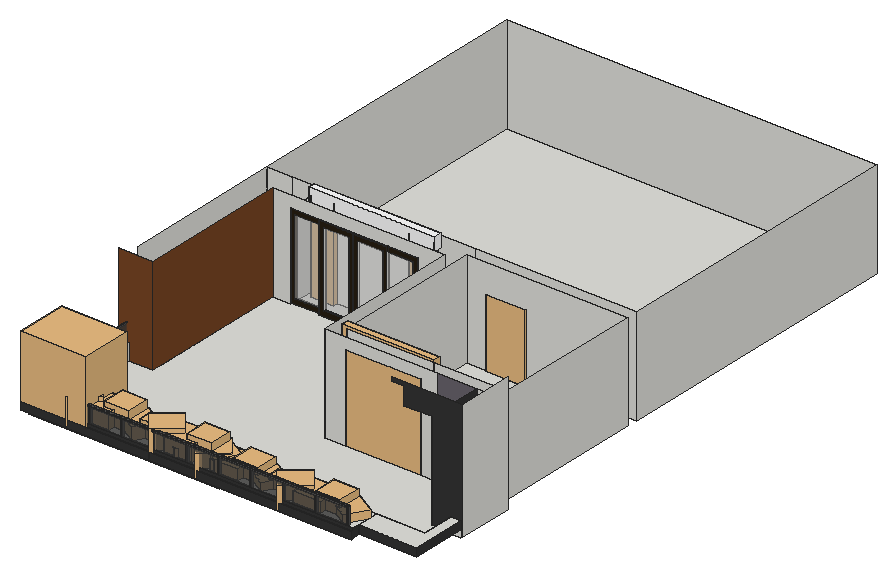
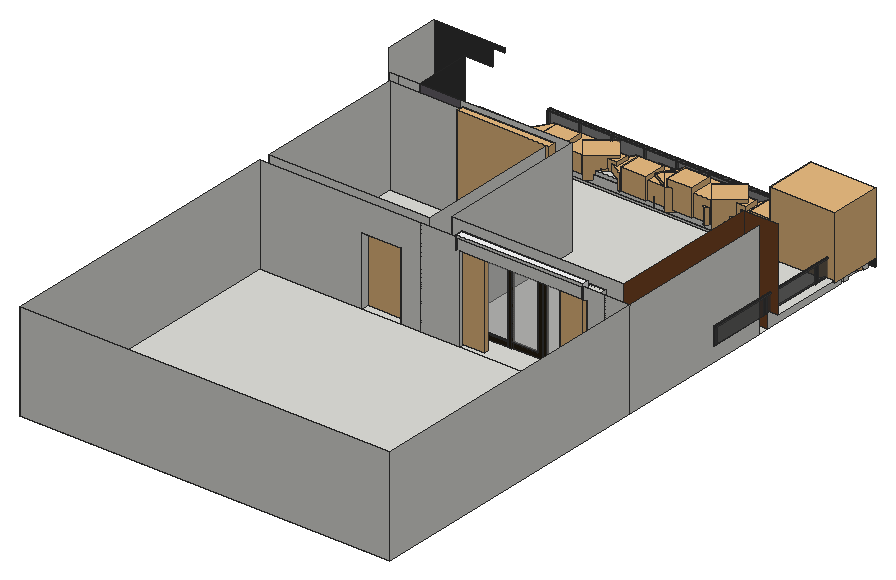
# SketchUp Ruby script. Lengths in inches.
U = 1.inch
M = Sketchup.active_model
def pt(a) = Geom::Point3d.new(a.map { |v| v * U })
def face(e, loops, mat)
  f = e.add_face(loops[0].map { |a| pt(a) })
  loops[1..].each { |l| e.add_face(l.map { |a| pt(a) }).erase! }
  f.material = f.back_material = mat if mat
  f
end
# faces: each face lists its corners as indices into pts; further lists are holes
def faces(e, pts, list, mat = nil) = list.each { |f| face(e, (f[0].is_a?(Array) ? f : [f]).map { |l| l.map { |i| pts[i] } }, mat) }
# xy, xz, yz: faces in a plane at the given z, y or x. An outline is a flat list of corners, or four numbers for a rectangle; further outlines are holes
def ring(l) = l.size == 4 ? [[l[0], l[1]], [l[2], l[1]], [l[2], l[3]], [l[0], l[3]]] : l.each_slice(2).to_a
def flat(e, list, mat, &to3) = list.each { |f| face(e, (f[0].is_a?(Array) ? f : [f]).map { |l| ring(l).map { |u, v| to3.(u, v) } }, mat) }
def xy(e, z, list, mat = nil) = flat(e, list, mat) { |x, y| [x, y, z] }
def xz(e, y, list, mat = nil) = flat(e, list, mat) { |x, z| [x, y, z] }
def yz(e, x, list, mat = nil) = flat(e, list, mat) { |y, z| [x, y, z] }
def lines(e, pts, list) = list.each { |a, b| e.add_line(pt(pts[a]), pt(pts[b])) }
# prism: a flat outline (further loops are holes) pulled along v
def prism(e, loops, v, mat = nil)
  f = face(e, loops, mat); d = Geom::Vector3d.new(v.map { |x| x * U })
  f.pushpull(f.normal.samedirection?(d) ? d.length : -d.length)
end
def box(e, o, s, mat = nil) = prism(e, [[o, [o[0] + s[0], o[1], o[2]], [o[0] + s[0], o[1] + s[1], o[2]], [o[0], o[1] + s[1], o[2]]]], [0, 0, s[2]], mat)
def at(x, y, z, deg = 0) = Geom::Transformation.translation(pt([x, y, z])) * Geom::Transformation.rotation(ORIGIN, Z_AXIS, deg.degrees)
def axes(o, x, y, z) = Geom::Transformation.new([*x, 0, *y, 0, *z, 0, *pt(o).to_a, 1])
def part(name) = M.definitions.add(name)
# library, detail: a bought-in or finely detailed component or shape, given as its bounding box
def library(name, o, s) = part(name).tap { |d| box(d.entities, o, s) }
def detail(e, o, s) = box(e.add_group.entities, o, s)
def put(e, d, t, mat = nil) = e.add_instance(d, t).tap { |i| i.material = mat if mat }
def group(e, t, mat = nil) = e.add_group.tap { |g| g.transformation = t; g.material = mat if mat }.entities
root = M.entities
M.materials.add("DefaultMaterial4").color = [255, 255, 255]
M.materials.add("Material__1").color = [95, 70, 46]
M.materials.add("[0135_DarkGray]").color = [81, 81, 81]
M.materials.add("[Color M07]").color = [53, 53, 53]
M.materials.add("[Slate Light Tile]").color = [105, 101, 109]
M.materials.add("[Translucent Glass Gray]2").color = [201, 201, 201]
M.materials["[Translucent Glass Gray]2"].alpha = 0.5
M.materials.add("[Translucent Glass Safety]").color = [204, 235, 244]
M.materials["[Translucent Glass Safety]"].alpha = 0.5
M.materials.add("[Translucent_Glass_Gray]1").color = [63, 63, 63]
M.materials["[Translucent_Glass_Gray]1"].alpha = 0.54
M.materials.add("[Wood Veneer 01]").color = [120, 70, 37]
M.materials.add("curtain").color = [207, 207, 207]
M.materials["curtain"].alpha = 0.74
M.materials.add("oak swatch").color = [40, 31, 19]
c1 = library("Group\#21",[-0.5,-0.5,0],[11,185.21,2.6875])
c2 = library("Mesh Light\#2",[-0.5,-0.5,-0.1],[1,1,0.2])
c3 = library("Group\#22",[-0.5,-0.5,-0.1],[11,185.21,0.2])
c4 = library("Group\#20",[-0.5,-0.5,-0.1],[11,185.21,0.2])
c5 = library("元件\#5",[-4.39,0,0],[5.37,35.83,90.55])
c6 = library("Sliding Door",[0,0,0],[94.49,5.83,91.73])
c7 = part("Group\#1")
box(c7.entities,[0,0,0],[1.77,4.72,80.31],"oak swatch")
c8 = part("Exterior Sliding Doors")
xy(c8.entities,0,[[1.77,33.07,3.54,70.87],[1.77,70.87,3.54,108.66]])
xy(c8.entities,0,[[0,0,1.77,33.07],[0,108.66,1.77,141.73]],"oak swatch")
xy(c8.entities,4.72,[[0,4.72,1.77,33.07],[1.77,37.8,3.54,66.14],[1.77,75.88,3.54,103.9375],[0,108.66,1.77,137.01]],"oak swatch")
xy(c8.entities,75.59,[[1.77,37.8,3.54,66.14],[1.77,75.88,3.54,103.9375]])
xy(c8.entities,75.59,[[0,4.72,1.77,33.07],[0,108.66,1.77,137.01]],"oak swatch")
xy(c8.entities,80.31,[[0,0,1.77,33.07],[1.77,33.07,3.54,70.87],[1.77,70.87,3.54,108.66],[0,108.66,1.77,141.73]],"oak swatch")
xz(c8.entities,0,[[0,0,1.77,80.31]],"oak swatch")
xz(c8.entities,4.72,[[0,4.72,1.77,75.59]],"oak swatch")
xz(c8.entities,33.07,[[0,0,1.77,4.72],[1.77,0,3.54,80.31],[0,75.59,1.77,80.31]],"oak swatch")
xz(c8.entities,37.8,[[1.77,4.72,3.54,75.59]])
xz(c8.entities,66.14,[[1.77,4.72,3.54,75.59]],"oak swatch")
xz(c8.entities,70.87,[[1.77,0,3.54,80.31]])
xz(c8.entities,75.88,[[1.77,4.72,3.54,75.59]])
xz(c8.entities,103.9375,[[1.77,4.72,3.54,75.59]],"oak swatch")
xz(c8.entities,108.66,[[1.77,4.72,3.54,75.59]])
xz(c8.entities,108.66,[[0,0,3.54,4.72],[0,75.59,3.54,80.31]],"oak swatch")
xz(c8.entities,137.01,[[0,4.72,1.77,75.59]],"oak swatch")
xz(c8.entities,141.73,[[0,0,1.77,80.31]],"oak swatch")
yz(c8.entities,0,[[0,0,33.07,0,33.07,4.72,4.72,4.72,4.72,75.59,33.07,75.59,33.07,80.31,0,80.31],[108.66,0,141.73,0,141.73,80.31,108.66,80.31,108.66,75.59,137.01,75.59,137.01,4.72,108.66,4.72]],"oak swatch")
yz(c8.entities,1.77,[[4.72,4.72,33.07,75.59],[37.8,4.72,66.14,75.59],[75.88,4.72,103.9375,75.59],[108.66,4.72,137.01,75.59]],"[Translucent Glass Gray]2")
yz(c8.entities,1.77,[[0,0,33.07,0,33.07,4.72,4.72,4.72,4.72,75.59,33.07,75.59,33.07,80.31,0,80.31],[[33.07,0,70.87,80.31],[37.8,4.72,66.14,75.59]],[[70.87,0,141.73,80.31],[108.66,4.72,137.01,75.59],[75.88,4.72,103.9375,75.59]]],"oak swatch")
yz(c8.entities,3.54,[[[33.07,0,70.87,80.31],[37.8,4.72,66.14,75.59]],[[70.87,0,108.66,80.31],[75.88,4.72,103.9375,75.59]]],"oak swatch")
put(c8.entities,c7,at(0,33.07,0))
put(c8.entities,c7,at(0,103.9375,0))
c9 = library("Plane02",[0.84,-3.92,-95.52],[32.2,7.84,95.63])
c10 = library("Window curtains",[0,0,0],[5.91,79.92,51.3])
c11 = library("Areca palm plant",[0,0,0],[49.1,36.6,54.46])
c12 = library("Group38\#2",[14.01,28.44,-23.43],[18.58,18.32,38.89])
c13 = library("Group\#32",[-84.69,-90.07,-0.36],[176.51,175.13,171.4])
c14 = library("Group20\#1",[-20.81,-17.08,3.79],[39.86,39.43,37.51])
c15 = library("Group\#130",[-7.34,-1.2,0],[38.67,35.81,49.04])
c16 = part("Group\#35")
put(c16.entities,c11,axes([-6.2,158.41,6.08],[0.45017,-0.56191,0],[0.66137,0.52986,0],[0,0,0.72]))
put(c16.entities,c11,axes([-6.2,56.6,6.08],[0.45017,-0.56191,0],[0.66137,0.52986,0],[0,0,0.72]))
put(c16.entities,c12,axes([-4.1,-1.15,28.17],[0.8848,0,0],[0,0.94674,0],[0,0,0.85826]))
put(c16.entities,c12,axes([-4.1,100.66,28.17],[0.8848,0,0],[0,0.94674,0],[0,0,0.85826]))
g1 = group(c16.entities,at(0,0,0))
xy(g1,0,[[0,0,6,234.8],[30,0,36,234.8]])
xy(g1,3,[[6,0,30,234.8]])
xy(g1,7,[[6,5,30,229.8]],"Material__1")
xy(g1,15,[[[0,0,36,234.8],[6,5,30,229.8]]])
xz(g1,0,[[0,0,6,0,6,3,30,3,30,0,36,0,36,15,0,15]])
xz(g1,5,[[6,7,30,15]])
xz(g1,229.8,[[6,7,30,15]])
xz(g1,234.8,[[0,0,0,15,36,15,36,0,30,0,30,3,6,3,6,0]])
yz(g1,0,[[0,0,234.8,15]])
yz(g1,6,[[0,0,234.8,3],[5,7,229.8,15]])
yz(g1,30,[[0,0,234.8,3],[5,7,229.8,15]])
yz(g1,36,[[0,0,234.8,15]])
put(c16.entities,c13,axes([17.19,121.23,6.07],[-0.08133,-0.14087,0],[0.14087,-0.08133,0],[0,0,0.1725]))
put(c16.entities,c13,axes([14.93,173.12,6.05],[-0.04961,-0.08593,0],[0.08593,-0.04961,0],[0,0,0.10522]))
put(c16.entities,c14,axes([18.97,79.98,4.77],[0,0.85,0],[-0.85,0,0],[0,0,0.85]))
put(c16.entities,c13,axes([17.19,223.04,6.07],[-0.08133,-0.14087,0],[0.14087,-0.08133,0],[0,0,0.1725]))
put(c16.entities,c13,axes([14.93,71.3,6.05],[-0.04961,-0.08593,0],[0.08593,-0.04961,0],[0,0,0.10522]))
put(c16.entities,c15,axes([24.9375,191.72,8],[0,0.79,0],[-0.79,0,0],[0,0,0.79]))
put(c16.entities,c14,axes([18.97,181.79,4.77],[0,0.85,0],[-0.85,0,0],[0,0,0.85]))
put(c16.entities,c15,axes([24.9375,89.91,8],[0,0.79,0],[-0.79,0,0],[0,0,0.79]))
put(c16.entities,c13,axes([14.93,91.37,6.05],[-0.04961,-0.08593,0],[0.08593,-0.04961,0],[0,0,0.10522]))
put(c16.entities,c13,axes([14.93,145.87,6.05],[-0.04961,-0.08593,0],[0.08593,-0.04961,0],[0,0,0.10522]))
put(c16.entities,c13,axes([17.19,15.79,6.07],[-0.08133,-0.14087,0],[0.14087,-0.08133,0],[0,0,0.1725]))
put(c16.entities,c13,axes([14.93,193.18,6.05],[-0.04961,-0.08593,0],[0.08593,-0.04961,0],[0,0,0.10522]))
put(c16.entities,c13,axes([14.93,44.05,6.05],[-0.04961,-0.08593,0],[0.08593,-0.04961,0],[0,0,0.10522]))
c17 = library("Round Planter with Plant",[-35.48,-39.77,0],[80.62,63.55,77.875])
c18 = part("Group\#81")
box(c18.entities,[0,0,0],[0.79,39.37,35.43],"[Translucent_Glass_Gray]1")
c19 = part("Group\#82")
box(c19.entities,[0,0,0],[0.59,1.57,34.25])
c20 = part("Group\#85")
g2 = group(c20.entities,at(0.55,0.5,0))
put(g2,c18,axes([293.06,0,0],[0,0.84,0],[-0.92977,0,0],[0,0,1]),"[Translucent Glass Safety]")
g3 = group(g2,at(0,33.57,0),"[Translucent Glass Safety]")
box(g3,[0,0,0],[0.73,33.07,35.43],"[Translucent_Glass_Gray]1")
put(g2,c18,axes([218.38,0,0],[0,0.84,0],[-0.92977,0,0],[0,0,1]),"[Translucent Glass Safety]")
put(g2,c18,axes([367.73,0,0],[0,0.84,0],[-0.92977,0,0],[0,0,1]),"[Translucent Glass Safety]")
g4 = group(g2,at(31.69,0,0),"[Translucent Glass Safety]")
box(g4,[-30.96,0,0],[30.96,0.66,35.43],"[Translucent_Glass_Gray]1")
put(g2,c18,axes([255.72,0,0],[0,0.84,0],[-0.92977,0,0],[0,0,1]),"[Translucent Glass Safety]")
g5 = group(g2,at(181.04,0,0),"[Translucent Glass Safety]")
box(g5,[-36.61,0,0],[36.61,0.66,35.43],"[Translucent_Glass_Gray]1")
g6 = group(g2,at(0,0.66,0),"[Translucent Glass Safety]")
box(g6,[0,0,0],[0.73,32.24,35.43],"[Translucent_Glass_Gray]1")
g7 = group(g2,at(143.71,0,0),"[Translucent Glass Safety]")
box(g7,[-36.61,0,0],[36.61,0.66,35.43],"[Translucent_Glass_Gray]1")
g8 = group(g2,at(69.03,0,0),"[Translucent Glass Safety]")
box(g8,[-36.61,0,0],[36.61,0.66,35.43],"[Translucent_Glass_Gray]1")
g9 = group(g2,at(0,67.3,0),"[Translucent Glass Safety]")
box(g9,[0,0,0],[0.73,33.07,35.43],"[Translucent_Glass_Gray]1")
put(g2,c19,axes([107.44,0.66,0],[0,1,0],[-0.92977,0,0],[0,0,1]),"[0135_DarkGray]")
put(g2,c19,axes([144.78,0.66,0],[0,1,0],[-0.92977,0,0],[0,0,1]),"[0135_DarkGray]")
put(g2,c19,axes([182.11,0.66,0],[0,1,0],[-0.92977,0,0],[0,0,1]),"[0135_DarkGray]")
put(g2,c19,axes([256.79,0.66,0],[0,1,0],[-0.92977,0,0],[0,0,1]),"[0135_DarkGray]")
put(g2,c19,axes([368.14,0.66,0],[0,1,0],[-0.92977,0,0],[0,0,1]),"[0135_DarkGray]")
put(g2,c19,axes([0.73,98.83,0],[0.92977,0,0],[0,1,0],[0,0,1]),"[0135_DarkGray]")
put(g2,c19,axes([331.46,0.66,0],[0,1,0],[-0.92977,0,0],[0,0,1]),"[0135_DarkGray]")
g10 = group(g2,at(106.37,0,0),"[Translucent Glass Safety]")
box(g10,[-36.61,0,0],[36.61,0.66,35.43],"[Translucent_Glass_Gray]1")
put(g2,c18,axes([330.39,0,0],[0,0.84,0],[-0.92977,0,0],[0,0,1]),"[Translucent Glass Safety]")
put(g2,c19,axes([294.125,0.66,0],[0,1,0],[-0.92977,0,0],[0,0,1]),"[0135_DarkGray]")
put(g2,c19,axes([0.73,66.04,0],[0.92977,0,0],[0,1,0],[0,0,1]),"[0135_DarkGray]")
put(g2,c19,axes([0.73,32.31,0],[0.92977,0,0],[0,1,0],[0,0,1]),"[0135_DarkGray]")
put(g2,c19,axes([32.76,0.66,0],[0,1,0],[-0.92977,0,0],[0,0,1]),"[0135_DarkGray]")
put(g2,c19,axes([70.1,0.66,0],[0,1,0],[-0.92977,0,0],[0,0,1]),"[0135_DarkGray]")
put(g2,c19,axes([219.45,0.66,0],[0,1,0],[-0.92977,0,0],[0,0,1]),"[0135_DarkGray]")
g11 = group(c20.entities,at(0,0,34.25))
xy(g11,0,[[0,0,0,100.87,0.55,100.87,0.55,0.5,362.73,0.5,362.73,0],[362.73,0,369.35,0.5],[368.19,0.5,368.6875,1.16],[1.28,1.16,1.28,100.87,1.83,100.87,1.83,1.65,362.73,1.65,362.73,1.16],[362.73,1.16,368.19,1.65]],"[0135_DarkGray]")
xy(g11,1.18,[[368.19,0,368.6875,0.5],[368.6875,0,369.35,0.5],[0.55,0.5,0.55,100.87,1.28,100.87,1.28,1.16,362.73,1.16,362.73,0.5],[368.6875,0.5,369.35,1.16]],"[0135_DarkGray]")
xy(g11,1.97,[[0,0,362.73,0,362.73,1.65,1.83,1.65,1.83,100.87,0,100.87],[362.73,0,368.19,1.65]],"[0135_DarkGray]")
xz(g11,0,[[0,0,362.73,1.97],[362.73,0,369.35,0,369.35,1.18,368.19,1.18,368.19,1.97,362.73,1.97]],"[0135_DarkGray]")
xz(g11,0.5,[[0.55,0,1.28,1.18],[1.28,0,362.73,1.18],[362.73,0,368.19,1.18],[368.19,0,368.6875,1.18],[368.6875,0,369.35,1.18]],"[0135_DarkGray]")
xz(g11,1.16,[[1.28,0,362.73,1.18],[362.73,0,368.19,1.18]],"[0135_DarkGray]")
xz(g11,1.65,[[1.83,0,362.73,1.97],[362.73,0,368.19,1.97]],"[0135_DarkGray]")
xz(g11,100.87,[[0,0,0,1.97,1.83,1.97,1.83,0,1.28,0,1.28,1.18,0.55,1.18,0.55,0]],"[0135_DarkGray]")
yz(g11,0,[[0,0,100.87,1.97]],"[0135_DarkGray]")
yz(g11,0.55,[[0.5,0,100.87,1.18]],"[0135_DarkGray]")
yz(g11,1.28,[[1.16,0,100.87,1.18]],"[0135_DarkGray]")
yz(g11,1.83,[[1.65,0,100.87,1.97]],"[0135_DarkGray]")
yz(g11,362.73,[[0,0,0,1.97,1.65,1.97,1.65,0,1.16,0,1.16,1.18,0.5,1.18,0.5,0]],"[0135_DarkGray]")
yz(g11,368.19,[[1.16,0,1.65,0,1.65,1.97,0,1.97,0,1.18,1.16,1.18],[0.5,0,1.16,1.18]],"[0135_DarkGray]")
yz(g11,368.6875,[[0.5,0,1.16,1.18]],"[0135_DarkGray]")
yz(g11,369.35,[[0,0,0.5,1.18]],"[0135_DarkGray]")
c21 = library("Spot Light",[-5.1,-5.1,-11.05],[10.2,10.2,11.05])
c22 = part("Group\#68")
xy(c22.entities,48.43,[[59.06,0,59.06,5.91,59.65,5.91,59.65,0.59,138.39,0.59,138.39,5.91,138.98,5.91,138.98,0]],"DefaultMaterial4")
xy(c22.entities,53.9375,[[59.65,0.59,138.39,5.91]],"DefaultMaterial4")
xy(c22.entities,55.51,[[59.06,0,138.98,5.91]],"DefaultMaterial4")
xz(c22.entities,0,[[59.06,48.43,138.98,55.51]],"DefaultMaterial4")
xz(c22.entities,0.59,[[59.65,48.43,138.39,53.9375]],"DefaultMaterial4")
xz(c22.entities,5.91,[[59.06,48.43,59.06,55.51,138.98,55.51,138.98,48.43,138.39,48.43,138.39,53.9375,59.65,53.9375,59.65,48.43]])
yz(c22.entities,59.06,[[0,48.43,5.91,55.51]],"DefaultMaterial4")
yz(c22.entities,138.39,[[0.59,48.43,5.91,53.9375]],"DefaultMaterial4")
yz(c22.entities,138.98,[[0,48.43,5.91,55.51]],"DefaultMaterial4")
xy(root,132,[[190.19,395.75,645.31,395.75,645.31,438.56,619.25,438.56,619.25,508.37,550.28,508.37,550.28,522.1,457.97,522.1,457.97,508.37,431.89,508.37,431.89,692.93,399.32,692.93,399.32,721.37,242.57,721.37,242.57,692.93,220.4375,692.93,220.4375,508.37,190.19,508.37],[645.31,436.28,657.75,438.56],[619.25,438.56,657.75,508.37],[190.19,508.37,220.4375,522.1],[190.19,522.1,220.4375,522.1,220.4375,692.93,220.5,692.93,220.5,721.37,190.19,721.37],
  [447.875,522.1,645.31,522.1,645.31,707.71,519.83,707.71,519.83,721.37,471.83,721.37,471.83,707.71,447.875,707.71],[190.19,721.37,645.31,1090.87]])
xy(root,139.1,[[177.75,357.25,585.62,359.375]])
xy(root,141.4375,[[585.62,368.125,585.62,395.75,645.31,395.75,645.31,436.28,657.75,436.28,657.75,368.125]])
xy(root,148.36,[[177.75,357.25,585.62,359.375]])
xy(root,151.5,[[177.75,359.375,585.62,359.375,585.62,395.75,190.19,395.75,190.19,508.37,177.75,508.37],[585.62,368.125,657.75,368.125,657.75,436.28,645.31,436.28,645.31,395.75,585.62,395.75]])
xy(root,195.89,[[590.91,497.87,596.29,508.37]])
xy(root,212.71,[[590.91,497.87,596.29,508.37]])
xy(root,216,[[471.83,707.71,519.83,721.37]])
xy(root,237.9375,[[242.57,692.93,399.32,721.37]])
xy(root,238.0625,[[457.97,508.37,550.28,522.1]])
xz(root,357.25,[[177.75,139.1,585.62,148.36]],"[Color M07]")
xz(root,359.375,[[177.75,148.36,585.62,151.5]],"[Color M07]")
xz(root,368.125,[[585.62,141.4375,657.75,151.5]],"[Color M07]")
xz(root,395.75,[[190.19,132,585.62,151.5],[585.62,132,645.31,141.4375],[585.62,141.4375,645.31,151.5]])
xz(root,436.28,[[645.31,132,657.75,141.4375],[645.31,141.4375,657.75,151.5]])
xz(root,438.56,[[619.25,132,657.75,132,657.75,278.125,569.82,278.125,569.82,273.1875,585.62,273.1875,585.62,252,619.25,252]],"[Color M07]")
xz(root,497.87,[[590.91,195.89,596.29,212.71]])
xz(root,508.37,[[431.89,132,457.97,132,457.97,238.0625,550.28,238.0625,550.28,132,569.82,132,569.82,252,431.89,252],[619.25,132,645.31,252],[645.31,132,657.75,252]])
xz(root,508.37,[[[569.82,132,619.25,252],[590.91,195.89,596.29,212.71]]],"[Slate Light Tile]")
xz(root,508.37,[[190.19,132,220.4375,132,220.4375,252,177.75,252,177.75,151.5,190.19,151.5]],"[Wood Veneer 01]")
xz(root,522.1,[[447.875,132,447.875,252,645.31,252,645.31,132,550.28,132,550.28,238.0625,457.97,238.0625,457.97,132]])
xz(root,692.93,[[220.4375,132,242.57,132,242.57,237.9375,399.32,237.9375,399.32,132,431.89,132,431.89,252,220.4375,252]])
xz(root,707.71,[[447.875,132,471.83,132,471.83,216,519.83,216,519.83,132,645.31,132,645.31,252,447.875,252]])
xz(root,721.37,[[190.19,132,220.5,252],[220.5,132,220.5,252,447.875,252,447.875,132,399.32,132,399.32,237.9375,242.57,237.9375,242.57,132],[447.875,132,447.875,252,645.31,252,645.31,132,519.83,132,519.83,216,471.83,216,471.83,132]])
xz(root,1090.87,[[190.19,132,645.31,252]])
yz(root,190.19,[[395.75,132,508.37,151.5],[522.1,132,721.37,252],[721.37,132,1090.87,252]])
yz(root,220.4375,[[508.37,132,692.93,252]],"[Wood Veneer 01]")
yz(root,242.57,[[692.93,132,721.37,237.9375]])
yz(root,399.32,[[692.93,132,721.37,237.9375]])
yz(root,431.89,[[508.37,132,692.93,252]])
yz(root,447.875,[[522.1,132,707.71,252]])
yz(root,457.97,[[508.37,132,522.1,238.0625]])
yz(root,471.83,[[707.71,132,721.37,216]])
yz(root,519.83,[[707.71,132,721.37,216]])
yz(root,550.28,[[508.37,132,522.1,238.0625]])
yz(root,585.62,[[368.125,141.4375,395.75,151.5]])
yz(root,585.62,[[357.25,139.1,359.375,139.1,368.125,141.4375,368.125,151.5,359.375,151.5,359.375,148.36,357.25,148.36]],"[Color M07]")
yz(root,590.91,[[497.87,195.89,508.37,212.71]])
yz(root,596.29,[[497.87,195.89,508.37,212.71]])
yz(root,619.25,[[438.56,132,508.37,252]],"[Color M07]")
yz(root,645.31,[[395.75,132,436.28,141.4375],[522.1,132,707.71,252],[721.37,132,1090.87,252],[395.75,141.4375,436.28,151.5]])
yz(root,657.75,[[438.56,132,508.37,278.125]])
yz(root,657.75,[[368.125,141.4375,436.28,151.5]],"[Color M07]")
p = [[496.4,385.12,126],[495.11,385.29,126],[495.11,385.29,128.6875],[496.4,385.12,128.6875],[497.69,385.29,126],[497.69,385.29,128.6875],
  [552.71,385.12,126],[551.42,385.29,126],[551.42,385.29,128.6875],[552.71,385.12,128.6875],[554.01,385.29,126],[554.01,385.29,128.6875],
  [493.9,385.79,126],[493.9,385.79,128.6875],[498.9,385.79,126],[498.9,385.79,128.6875],[550.21,385.79,126],[550.21,385.79,128.6875],
  [555.21,385.79,126],[555.21,385.79,128.6875],[492.86,386.58,126],[492.86,386.58,128.6875],[499.93,386.58,126],[499.93,386.58,128.6875],
  [549.18,386.58,126],[549.18,386.58,128.6875],[556.25,386.58,126],[556.25,386.58,128.6875],[492.07,387.62,126],[492.07,387.62,128.6875],
  [500.73,387.62,126],[500.73,387.62,128.6875],[548.38,387.62,126],[548.38,387.62,128.6875],[557.04,387.62,126],[557.04,387.62,128.6875],
  [491.57,388.83,126],[491.57,388.83,128.6875],[501.23,388.83,126],[501.23,388.83,128.6875],[547.88,388.83,126],[547.88,388.83,128.6875],
  [557.54,388.83,126],[557.54,388.83,128.6875],[491.4,390.12,126],[491.4,390.12,128.6875],[501.4,390.12,126],[501.4,390.12,128.6875],
  [547.71,390.12,126],[547.71,390.12,128.6875],[557.71,390.12,126],[557.71,390.12,128.6875],[491.57,391.41,126],[491.57,391.41,128.6875],
  [501.23,391.41,126],[501.23,391.41,128.6875],[547.88,391.41,126],[547.88,391.41,128.6875],[557.54,391.41,126],[557.54,391.41,128.6875],
  [492.07,392.62,126],[492.07,392.62,128.6875],[500.73,392.62,126],[500.73,392.62,128.6875],[548.38,392.62,126],[548.38,392.62,128.6875],
  [557.04,392.62,126],[557.04,392.62,128.6875],[492.86,393.66,126],[492.86,393.66,128.6875],[499.93,393.66,126],[499.93,393.66,128.6875],
  [549.18,393.66,126],[549.18,393.66,128.6875],[556.25,393.66,126],[556.25,393.66,128.6875],[493.9,394.45,126],[493.9,394.45,128.6875],
  [498.9,394.45,126],[498.9,394.45,128.6875],[550.21,394.45,126],[550.21,394.45,128.6875],[555.21,394.45,126],[555.21,394.45,128.6875],
  [495.11,394.95,126],[495.11,394.95,128.6875],[497.69,394.95,126],[497.69,394.95,128.6875],[551.42,394.95,126],[551.42,394.95,128.6875],
  [554.01,394.95,126],[554.01,394.95,128.6875],[496.4,395.12,126],[496.4,395.12,128.6875],[552.71,395.12,126],[552.71,395.12,128.6875],
  [552.71,439.5625,126],[551.42,439.73,126],[551.42,439.73,128.6875],[552.71,439.5625,128.6875],[554.01,439.73,126],[554.01,439.73,128.6875],
  [550.21,440.23,126],[550.21,440.23,128.6875],[555.21,440.23,126],[555.21,440.23,128.6875],[549.18,441.03,126],[549.18,441.03,128.6875],
  [556.25,441.03,126],[556.25,441.03,128.6875],[548.38,442.0625,126],[548.38,442.0625,128.6875],[557.04,442.0625,126],[557.04,442.0625,128.6875],
  [547.88,443.27,126],[547.88,443.27,128.6875],[557.54,443.27,126],[557.54,443.27,128.6875],[547.71,444.5625,126],[547.71,444.5625,128.6875],
  [557.71,444.5625,126],[557.71,444.5625,128.6875],[547.88,445.86,126],[547.88,445.86,128.6875],[557.54,445.86,126],[557.54,445.86,128.6875],
  [548.38,447.0625,126],[548.38,447.0625,128.6875],[557.04,447.0625,126],[557.04,447.0625,128.6875],[549.18,448.1,126],[549.18,448.1,128.6875],
  [556.25,448.1,126],[556.25,448.1,128.6875],[550.21,448.89,126],[550.21,448.89,128.6875],[555.21,448.89,126],[555.21,448.89,128.6875],
  [551.42,449.39,126],[551.42,449.39,128.6875],[554.01,449.39,126],[554.01,449.39,128.6875],[552.71,449.5625,126],[552.71,449.5625,128.6875],
  [552.71,500.05,126],[551.42,500.22,126],[551.42,500.22,128.6875],[552.71,500.05,128.6875],[554.01,500.22,126],[554.01,500.22,128.6875],
  [550.21,500.72,126],[550.21,500.72,128.6875],[555.21,500.72,126],[555.21,500.72,128.6875],[549.18,501.52,126],[549.18,501.52,128.6875],
  [556.25,501.52,126],[556.25,501.52,128.6875],[548.38,502.55,126],[548.38,502.55,128.6875],[557.04,502.55,126],[557.04,502.55,128.6875],
  [547.88,503.76,126],[547.88,503.76,128.6875],[557.54,503.76,126],[557.54,503.76,128.6875],[547.71,505.05,126],[547.71,505.05,128.6875],
  [557.71,505.05,126],[557.71,505.05,128.6875],[547.88,506.35,126],[547.88,506.35,128.6875],[557.54,506.35,126],[557.54,506.35,128.6875],
  [548.38,507.55,126],[548.38,507.55,128.6875],[557.04,507.55,126],[557.04,507.55,128.6875],[499.93,508.59,126],[500.73,507.55,126],
  [500.73,507.55,128.125],[499.93,508.59,128.125],[549.18,508.59,126],[549.18,508.59,128.6875],[556.25,508.59,126],[556.25,508.59,128.6875],
  [498.9,509.38,126],[498.9,509.38,128.125],[550.21,509.38,126],[550.21,509.38,128.6875],[555.21,509.38,126],[555.21,509.38,128.6875],
  [497.69,509.88,126],[497.69,509.88,128.125],[551.42,509.88,126],[551.42,509.88,128.6875],[554.01,509.88,126],[554.01,509.88,128.6875],
  [496.4,510.05,126],[496.4,510.05,128.125],[552.71,510.05,126],[552.71,510.05,128.6875],[552.71,559.33,126],[551.42,559.5,126],
  [551.42,559.5,128.6875],[552.71,559.33,128.6875],[554.01,559.5,126],[554.01,559.5,128.6875],[550.21,560,126],[550.21,560,128.6875],
  [555.21,560,126],[555.21,560,128.6875],[549.18,560.79,126],[549.18,560.79,128.6875],[556.25,560.79,126],[556.25,560.79,128.6875],
  [548.38,561.83,126],[548.38,561.83,128.6875],[557.04,561.83,126],[557.04,561.83,128.6875],[547.88,563.03,126],[547.88,563.03,128.6875],
  [557.54,563.03,126],[557.54,563.03,128.6875],[547.71,564.33,126],[547.71,564.33,128.6875],[557.71,564.33,126],[557.71,564.33,128.6875],
  [547.88,565.62,126],[547.88,565.62,128.6875],[557.54,565.62,126],[557.54,565.62,128.6875],[548.38,566.83,126],[548.38,566.83,128.6875],
  [557.04,566.83,126],[557.04,566.83,128.6875],[549.18,567.86,126],[549.18,567.86,128.6875],[556.25,567.86,126],[556.25,567.86,128.6875],
  [550.21,568.66,126],[550.21,568.66,128.6875],[555.21,568.66,126],[555.21,568.66,128.6875],[551.42,569.16,126],[551.42,569.16,128.6875],
  [554.01,569.16,126],[554.01,569.16,128.6875],[552.71,569.33,126],[552.71,569.33,128.6875],[212.34,672.9375,126],[211.3,673.73,126],
  [211.3,673.73,126.875],[212.34,672.9375,126.875],[268.65,672.9375,126],[267.61,673.73,126],[267.61,673.73,126.875],[268.65,672.9375,126.875],
  [210.51,674.77,126],[210.51,674.77,126.875],[266.82,674.77,126],[266.82,674.77,126.875],[210.01,675.97,126],[210.01,675.97,126.875],
  [266.32,675.97,126],[266.32,675.97,126.875],[209.84,677.27,126],[209.84,677.27,126.875],[266.15,677.27,126],[266.15,677.27,126.875],
  [210.01,678.5625,126],[210.01,678.5625,126.875],[266.32,678.5625,126],[266.32,678.5625,126.875],[210.51,679.77,126],[210.51,679.77,126.875],
  [266.82,679.77,126],[266.82,679.77,126.875],[211.3,680.8,126],[211.3,680.8,126.875],[267.61,680.8,126],[267.61,680.8,126.875],
  [380.24,680.8,126],[379.44,679.77,126],[378.94,678.5625,126],[378.77,677.27,126],[378.94,675.97,126],[379.44,674.77,126],
  [380.24,673.73,126],[381.27,672.9375,126],[436.55,680.8,126],[435.76,679.77,126],[435.26,678.5625,126],[435.09,677.27,126],
  [435.26,675.97,126],[435.76,674.77,126],[436.55,673.73,126],[437.59,672.9375,126],[492.86,680.8,126],[492.07,679.77,126],
  [491.57,678.5625,126],[491.4,677.27,126],[491.57,675.97,126],[492.07,674.77,126],[492.86,673.73,126],[493.9,672.9375,126],
  [549.18,680.8,126],[548.38,679.77,126],[547.88,678.5625,126],[547.71,677.27,126],[547.88,675.97,126],[548.38,674.77,126],
  [549.18,673.73,126],[550.21,672.9375,126]]
faces(root,p,[[0,1,2,3],[4,0,3,5],[6,7,8,9],[10,6,9,11],[1,12,13,2],[14,4,5,15],[7,16,17,8],[18,10,11,19],
  [12,20,21,13],[22,14,15,23],[16,24,25,17],[26,18,19,27],[20,28,29,21],[30,22,23,31],[24,32,33,25],[34,26,27,35],
  [28,36,37,29],[38,30,31,39],[32,40,41,33],[42,34,35,43],[36,44,45,37],[46,38,39,47],[40,48,49,41],[50,42,43,51],
  [44,52,53,45],[54,46,47,55],[48,56,57,49],[58,50,51,59],[52,60,61,53],[62,54,55,63],[56,64,65,57],[66,58,59,67],
  [60,68,69,61],[70,62,63,71],[64,72,73,65],[74,66,67,75],[68,76,77,69],[78,70,71,79],[72,80,81,73],[82,74,75,83],
  [76,84,85,77],[86,78,79,87],[80,88,89,81],[90,82,83,91],[84,92,93,85],[92,86,87,93],[88,94,95,89],[94,90,91,95],
  [96,97,98,99],[100,96,99,101],[97,102,103,98],[104,100,101,105],[102,106,107,103],[108,104,105,109],[106,110,111,107],[112,108,109,113],
  [110,114,115,111],[116,112,113,117],[114,118,119,115],[120,116,117,121],[118,122,123,119],[124,120,121,125],[122,126,127,123],[128,124,125,129],
  [126,130,131,127],[132,128,129,133],[130,134,135,131],[136,132,133,137],[134,138,139,135],[140,136,137,141],[138,142,143,139],[142,140,141,143],
  [144,145,146,147],[148,144,147,149],[145,150,151,146],[152,148,149,153],[150,154,155,151],[156,152,153,157],[154,158,159,155],[160,156,157,161],
  [158,162,163,159],[164,160,161,165],[162,166,167,163],[168,164,165,169],[166,170,171,167],[172,168,169,173],[170,174,175,171],[176,172,173,177],
  [178,179,180,181],[174,182,183,175],[184,176,177,185],[186,178,181,187],[182,188,189,183],[190,184,185,191],[192,186,187,193],[188,194,195,189],
  [196,190,191,197],[198,192,193,199],[194,200,201,195],[200,196,197,201],[202,203,204,205],[206,202,205,207],[203,208,209,204],[210,206,207,211],
  [208,212,213,209],[214,210,211,215],[212,216,217,213],[218,214,215,219],[216,220,221,217],[222,218,219,223],[220,224,225,221],[226,222,223,227],
  [224,228,229,225],[230,226,227,231],[228,232,233,229],[234,230,231,235],[232,236,237,233],[238,234,235,239],[236,240,241,237],[242,238,239,243],
  [240,244,245,241],[246,242,243,247],[244,248,249,245],[248,246,247,249],[250,251,252,253],[254,255,256,257],[251,258,259,252],[255,260,261,256],
  [258,262,263,259],[260,264,265,261],[262,266,267,263],[264,268,269,265],[266,270,271,267],[268,272,273,269],[270,274,275,271],[272,276,277,273],
  [274,278,279,275],[276,280,281,277]])
lines(root,p,[[282,283],[283,284],[284,285],[285,286],[286,287],[287,288],[288,289],[290,291],[291,292],[292,293],[293,294],[294,295],
  [295,296],[296,297],[298,299],[299,300],[300,301],[301,302],[302,303],[303,304],[304,305],[306,307],[307,308],[308,309],
  [309,310],[310,311],[311,312],[312,313]])
put(root,c1,at(491.4,385.12,126))
g12 = group(root,at(209.84,385.12,126.5))
xy(g12,0,[[61.3125,0,60.02,0.17,58.8125,0.67,57.78,1.46,56.98,2.5,56.48,3.71,56.3125,5,56.48,6.29,56.98,7.5,57.78,8.54,58.8125,9.33,60.02,9.83,61.3125,10,62.61,9.83,63.8125,9.33,64.85,8.54,65.64,7.5,66.14,6.29,66.3125,5,66.14,3.71,65.64,2.5,64.85,1.46,63.8125,0.67,62.61,0.17]])
xy(g12,0.375,[[5,0,3.71,0.17,2.5,0.67,1.46,1.46,0.67,2.5,0.17,3.71,0,5,0.17,6.29,0.67,7.5,1.46,8.54,2.5,9.33,3.71,9.83,5,10,6.29,9.83,7.5,9.33,8.54,8.54,9.33,7.5,9.83,6.29,10,5,9.83,3.71,9.33,2.5,8.54,1.46,7.5,0.67,6.29,0.17],[5,54.44,3.71,54.61,2.5,55.11,1.46,55.9,0.67,56.94,0.17,58.15,0,59.44,0.17,60.73,0.67,61.94,1.46,62.98,2.5,63.77,3.71,64.27,5,64.44,6.29,64.27,7.5,63.77,8.54,62.98,9.33,61.94,9.83,60.73,10,59.44,9.83,58.15,9.33,56.94,8.54,55.9,7.5,55.11,6.29,54.61],[61.3125,54.44,60.02,54.61,58.8125,55.11,57.78,55.9,56.98,56.94,56.48,58.15,56.3125,59.44,56.48,60.73,56.98,61.94,57.78,62.98,58.8125,63.77,60.02,64.27,61.3125,64.44,62.61,64.27,63.8125,63.77,64.85,62.98,65.64,61.94,66.14,60.73,66.3125,59.44,66.14,58.15,65.64,56.94,64.85,55.9,63.8125,55.11,62.61,54.61],[5,114.93,3.71,115.1,2.5,115.6,1.46,116.4,0.67,117.43,0.17,118.64,0,119.93,0.17,121.22,0.67,122.43,1.46,123.47,2.5,124.26,3.71,124.76,5,124.93,6.29,124.76,7.5,124.26,8.54,123.47,9.33,122.43,9.83,121.22,10,119.93,9.83,118.64,9.33,117.43,8.54,116.4,7.5,115.6,6.29,115.1],[61.3125,114.93,60.02,115.1,58.8125,115.6,57.78,116.4,56.98,117.43,56.48,118.64,56.3125,119.93,56.48,121.22,56.98,122.43,57.78,123.47,58.8125,124.26,60.02,124.76,61.3125,124.93,62.61,124.76,63.8125,124.26,64.85,123.47,65.64,122.43,66.14,121.22,66.3125,119.93,66.14,118.64,65.64,117.43,64.85,116.4,63.8125,115.6,62.61,115.1],
  [5,174.21,3.71,174.375,2.5,174.875,1.46,175.67,0.67,176.71,0.17,177.91,0,179.21,0.17,180.5,0.67,181.71,1.46,182.74,2.5,183.54,3.71,184.04,5,184.21,6.29,184.04,7.5,183.54,8.54,182.74,9.33,181.71,9.83,180.5,10,179.21,9.83,177.91,9.33,176.71,8.54,175.67,7.5,174.875,6.29,174.375],[61.3125,174.21,60.02,174.375,58.8125,174.875,57.78,175.67,56.98,176.71,56.48,177.91,56.3125,179.21,56.48,180.5,56.98,181.71,57.78,182.74,58.8125,183.54,60.02,184.04,61.3125,184.21,62.61,184.04,63.8125,183.54,64.85,182.74,65.64,181.71,66.14,180.5,66.3125,179.21,66.14,177.91,65.64,176.71,64.85,175.67,63.8125,174.875,62.61,174.375],[5,287.15,3.71,287.32,2.5,287.82,1.46,288.61,0.67,289.65,0.17,290.85,0,292.15,0.17,293.44,0.67,294.65,1.46,295.68,2.5,296.48,3.71,296.98,5,297.15,6.29,296.98,7.5,296.48,8.54,295.68,9.33,294.65,9.83,293.44,10,292.15,9.83,290.85,9.33,289.65,8.54,288.61,7.5,287.82,6.29,287.32],[61.3125,287.15,60.02,287.32,58.8125,287.82,57.78,288.61,56.98,289.65,56.48,290.85,56.3125,292.15,56.48,293.44,56.98,294.65,57.78,295.68,58.8125,296.48,60.02,296.98,61.3125,297.15,62.61,296.98,63.8125,296.48,64.85,295.68,65.64,294.65,66.14,293.44,66.3125,292.15,66.14,290.85,65.64,289.65,64.85,288.61,63.8125,287.82,62.61,287.32]])
xy(g12,1.625,[[121.375,0,120.08,0.17,118.875,0.67,117.84,1.46,117.04,2.5,116.55,3.71,116.375,5,116.55,6.29,117.04,7.5,117.84,8.54,118.875,9.33,120.08,9.83,121.375,10,122.67,9.83,123.875,9.33,124.91,8.54,125.71,7.5,126.2,6.29,126.375,5,126.2,3.71,125.71,2.5,124.91,1.46,123.875,0.67,122.67,0.17],[173.9375,0,172.64,0.17,171.4375,0.67,170.4,1.46,169.61,2.5,169.11,3.71,168.9375,5,169.11,6.29,169.61,7.5,170.4,8.54,171.4375,9.33,172.64,9.83,173.9375,10,175.23,9.83,176.4375,9.33,177.47,8.54,178.27,7.5,178.77,6.29,178.9375,5,178.77,3.71,178.27,2.5,177.47,1.46,176.4375,0.67,175.23,0.17],[121.375,54.44,120.08,54.61,118.875,55.11,117.84,55.9,117.04,56.94,116.55,58.15,116.375,59.44,116.55,60.73,117.04,61.94,117.84,62.98,118.875,63.77,120.08,64.27,121.375,64.44,122.67,64.27,123.875,63.77,124.91,62.98,125.71,61.94,126.2,60.73,126.375,59.44,126.2,58.15,125.71,56.94,124.91,55.9,123.875,55.11,122.67,54.61],[173.9375,54.44,172.64,54.61,171.4375,55.11,170.4,55.9,169.61,56.94,169.11,58.15,168.9375,59.44,169.11,60.73,169.61,61.94,170.4,62.98,171.4375,63.77,172.64,64.27,173.9375,64.44,175.23,64.27,176.4375,63.77,177.47,62.98,178.27,61.94,178.77,60.73,178.9375,59.44,178.77,58.15,178.27,56.94,177.47,55.9,176.4375,55.11,175.23,54.61],[121.375,114.93,120.08,115.1,118.875,115.6,117.84,116.4,117.04,117.43,116.55,118.64,116.375,119.93,116.55,121.22,117.04,122.43,117.84,123.47,118.875,124.26,120.08,124.76,121.375,124.93,122.67,124.76,123.875,124.26,124.91,123.47,125.71,122.43,126.2,121.22,126.375,119.93,126.2,118.64,125.71,117.43,124.91,116.4,123.875,115.6,122.67,115.1],
  [173.9375,114.93,172.64,115.1,171.4375,115.6,170.4,116.4,169.61,117.43,169.11,118.64,168.9375,119.93,169.11,121.22,169.61,122.43,170.4,123.47,171.4375,124.26,172.64,124.76,173.9375,124.93,175.23,124.76,176.4375,124.26,177.47,123.47,178.27,122.43,178.77,121.22,178.9375,119.93,178.77,118.64,178.27,117.43,177.47,116.4,176.4375,115.6,175.23,115.1],[121.375,174.21,120.08,174.375,118.875,174.875,117.84,175.67,117.04,176.71,116.55,177.91,116.375,179.21,116.55,180.5,117.04,181.71,117.84,182.74,118.875,183.54,120.08,184.04,121.375,184.21,122.67,184.04,123.875,183.54,124.91,182.74,125.71,181.71,126.2,180.5,126.375,179.21,126.2,177.91,125.71,176.71,124.91,175.67,123.875,174.875,122.67,174.375],[173.9375,174.21,172.64,174.375,171.4375,174.875,170.4,175.67,169.61,176.71,169.11,177.91,168.9375,179.21,169.11,180.5,169.61,181.71,170.4,182.74,171.4375,183.54,172.64,184.04,173.9375,184.21,175.23,184.04,176.4375,183.54,177.47,182.74,178.27,181.71,178.77,180.5,178.9375,179.21,178.77,177.91,178.27,176.71,177.47,175.67,176.4375,174.875,175.23,174.375]])
put(g12,c2,axes([89.47,148.57,0.8125],[179.9375,0,0],[0,298.14749,0],[0,0,2.625]))
put(root,c3,at(435.09,385.12,128.125))
put(root,c4,at(547.71,385.12,128.6875))
put(root,c5,axes([471.83,708.08,132],[0,-1,0],[1.33978,0,0],[0,0,0.92765]))
put(root,c6,axes([457.97,508.37,132],[0.97697,0,0],[0,0.79008,0],[0,0,1.15622]))
put(root,c8,axes([242.57,694.88,133.25],[0,-1.1,0],[1.1,0,0],[0,0,1.30346]))
put(root,c9,axes([280,715.84,246.98],[-0.88913,0,0],[0,0.67314,0],[0,0,1.185]),"curtain")
put(root,c10,axes([555.64,522.1,134.05],[0,1.4541,0],[-1.4224,0,0],[0,0,2.35232]))
put(root,c9,axes([403.54,715.84,247.46],[-0.97301,0,0],[0,0.67314,0],[0,0,1.185]),"curtain")
put(root,c16,axes([185.83,396.93,136.5],[0,-1,0],[1,0,0],[0,0,0.83712]))
put(root,c16,axes([344.39,396.93,136.5],[0,-1,0],[1,0,0],[0,0,0.68]))
put(root,c17,at(213.23,397.02,148.36))
put(root,c20,axes([186.34,358.22,151.5],[1.06496,0,0],[0,2.34,0],[0,0,0.61]))
put(root,c21,at(593.6,497.87,195.89))
put(root,c21,axes([593.6,497.87,212.71],[-1,0,0],[0,1,0],[0,0,-1]))
put(root,c22,axes([133.4375,712.78,123.89],[1.94849,0,0],[0,1.4541,0],[0,0,2.35232]))
